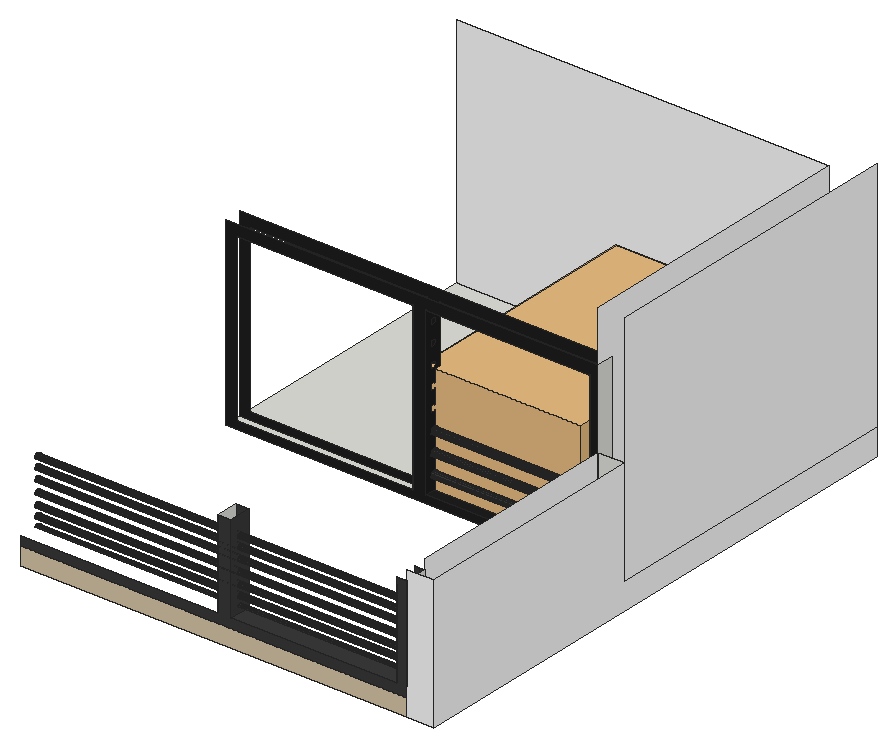
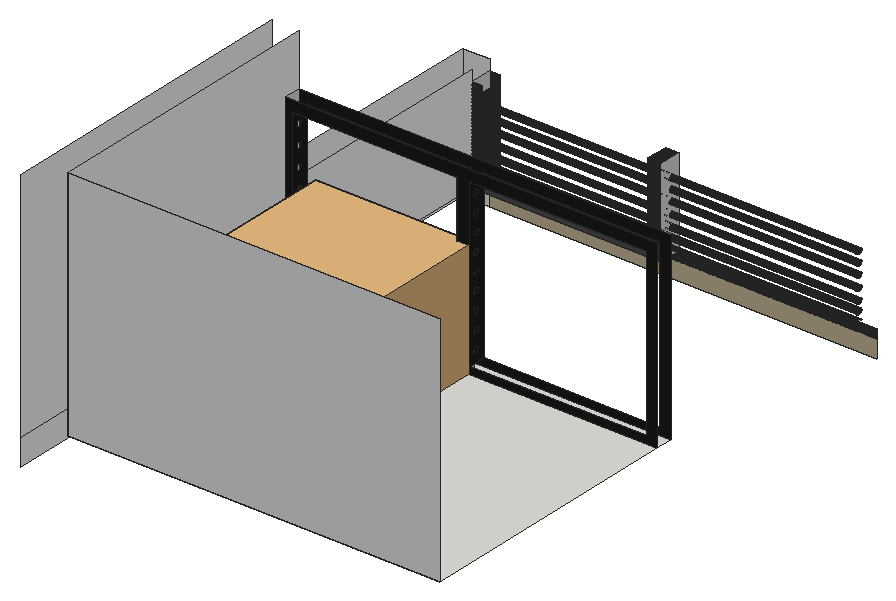
# SketchUp Ruby script. Lengths in inches.
U = 1.inch
M = Sketchup.active_model
def pt(a) = Geom::Point3d.new(a.map { |v| v * U })
def face(e, loops, mat)
  f = e.add_face(loops[0].map { |a| pt(a) })
  loops[1..].each { |l| e.add_face(l.map { |a| pt(a) }).erase! }
  f.material = f.back_material = mat if mat
  f
end
# faces: each face lists its corners as indices into pts; further lists are holes
def faces(e, pts, list, mat = nil) = list.each { |f| face(e, (f[0].is_a?(Array) ? f : [f]).map { |l| l.map { |i| pts[i] } }, mat) }
# xy, xz, yz: faces in a plane at the given z, y or x. An outline is a flat list of corners, or four numbers for a rectangle; further outlines are holes
def ring(l) = l.size == 4 ? [[l[0], l[1]], [l[2], l[1]], [l[2], l[3]], [l[0], l[3]]] : l.each_slice(2).to_a
def flat(e, list, mat, &to3) = list.each { |f| face(e, (f[0].is_a?(Array) ? f : [f]).map { |l| ring(l).map { |u, v| to3.(u, v) } }, mat) }
def xy(e, z, list, mat = nil) = flat(e, list, mat) { |x, y| [x, y, z] }
def xz(e, y, list, mat = nil) = flat(e, list, mat) { |x, z| [x, y, z] }
def yz(e, x, list, mat = nil) = flat(e, list, mat) { |y, z| [x, y, z] }
def lines(e, pts, list) = list.each { |a, b| e.add_line(pt(pts[a]), pt(pts[b])) }
# prism: a flat outline (further loops are holes) pulled along v
def prism(e, loops, v, mat = nil)
  f = face(e, loops, mat); d = Geom::Vector3d.new(v.map { |x| x * U })
  f.pushpull(f.normal.samedirection?(d) ? d.length : -d.length)
end
def box(e, o, s, mat = nil) = prism(e, [[o, [o[0] + s[0], o[1], o[2]], [o[0] + s[0], o[1] + s[1], o[2]], [o[0], o[1] + s[1], o[2]]]], [0, 0, s[2]], mat)
def at(x, y, z, deg = 0) = Geom::Transformation.translation(pt([x, y, z])) * Geom::Transformation.rotation(ORIGIN, Z_AXIS, deg.degrees)
def axes(o, x, y, z) = Geom::Transformation.new([*x, 0, *y, 0, *z, 0, *pt(o).to_a, 1])
def part(name) = M.definitions.add(name)
# library, detail: a bought-in or finely detailed component or shape, given as its bounding box
def library(name, o, s) = part(name).tap { |d| box(d.entities, o, s) }
def detail(e, o, s) = box(e.add_group.entities, o, s)
def put(e, d, t, mat = nil) = e.add_instance(d, t).tap { |i| i.material = mat if mat }
def group(e, t, mat = nil) = e.add_group.tap { |g| g.transformation = t; g.material = mat if mat }.entities
root = M.entities
M.materials.add("[Carrera Marble]").color = [252, 252, 252]
M.materials.add("[Color M07]").color = [58, 58, 58]
M.materials.add("[Color M08]").color = [30, 30, 30]
M.materials.add("[Field Square Tile]").color = [217, 201, 169]
M.materials.add("[Formica Laminate Dark]").color = [50, 53, 60]
c1 = library("2015 Porsche Macan",[0.14,0.6,0.32],[90.05,184.43,65.58])
xy(root,15.1875,[[467.61,406.29,679.23,416.16],[467.61,416.16,679.23,570.65]])
xy(root,15.1875,[[579.17,270.82,673.42,283.23]],"[Color M07]")
xy(root,19.3125,[[581.54,406.29,674.94,416.16]],"[Color M08]")
xz(root,270.82,[[679.23,0,694.52,75.25]],"[Carrera Marble]")
xz(root,270.82,[[459.28,9.82,679.23,9.82,679.23,69.375,673.42,69.375,673.42,15.1875,579.17,15.1875,579.17,65.34,571.61,65.34,571.61,15.1875,459.28,15.1875]],"[Color M07]")
xz(root,270.82,[[459.28,0,679.23,9.82]],"[Field Square Tile]")
xz(root,283.23,[[571.61,15.1875,579.17,65.34],[673.42,15.1875,675.77,69.375],[675.77,15.1875,679.23,69.375]],"[Color M07]")
xz(root,406.29,[[679.23,15.1875,694.52,75.25]])
xz(root,406.29,[[[467.61,15.1875,679.23,119.75],[473.77,19.3125,574.36,113.6],[581.54,19.3125,674.94,113.6]]],"[Color M08]")
xz(root,416.16,[[[467.61,15.1875,679.23,119.75],[473.77,19.3125,574.36,113.6],[581.54,19.3125,674.94,113.6]]],"[Color M08]")
xz(root,570.65,[[467.61,15.1875,679.23,149.125]],"[Carrera Marble]")
yz(root,571.61,[[270.82,15.1875,283.23,65.34]])
yz(root,574.36,[[[406.29,19.3125,416.16,113.6],[411.5,83.75,412,83.8125,412.47,84.01,412.87,84.32,413.18,84.72,413.37,85.18,413.4375,85.6875,413.37,86.1875,413.18,86.65,412.87,87.06,412.47,87.36,412,87.56,411.5,87.625,411,87.56,410.53,87.36,410.13,87.06,409.82,86.65,409.63,86.1875,409.5625,85.6875,409.63,85.18,409.82,84.72,410.13,84.32,410.53,84.01,411,83.8125],[411.5,73.75,412,73.8125,412.47,74.01,412.87,74.32,413.18,74.72,413.37,75.18,413.4375,75.6875,413.37,76.1875,413.18,76.65,412.87,77.06,412.47,77.36,412,77.56,411.5,77.625,411,77.56,410.53,77.36,410.13,77.06,409.82,76.65,409.63,76.1875,409.5625,75.6875,409.63,75.18,409.82,74.72,410.13,74.32,410.53,74.01,411,73.8125],[411.5,63.75,412,63.8125,412.47,64.01,412.87,64.32,413.18,64.72,413.37,65.18,413.4375,65.6875,413.37,66.1875,413.18,66.65,412.87,67.06,412.47,67.36,412,67.56,411.5,67.625,411,67.56,410.53,67.36,410.13,67.06,409.82,66.65,409.63,66.1875,409.5625,65.6875,409.63,65.18,409.82,64.72,410.13,64.32,410.53,64.01,411,63.8125],[411.5,53.75,412,53.8125,412.47,54.01,412.87,54.32,413.18,54.72,413.37,55.18,413.4375,55.6875,413.37,56.1875,413.18,56.65,412.87,57.06,412.47,57.36,412,57.56,411.5,57.625,411,57.56,410.53,57.36,410.13,57.06,409.82,56.65,409.63,56.1875,409.5625,55.6875,409.63,55.18,409.82,54.72,410.13,54.32,410.53,54.01,411,53.8125],[411.5,43.75,412,43.8125,412.47,44.01,412.87,44.32,413.18,44.72,413.37,45.18,413.4375,45.6875,413.37,46.1875,413.18,46.65,412.87,47.06,412.47,47.36,412,47.56,411.5,47.625,411,47.56,410.53,47.36,410.13,47.06,409.82,46.65,409.63,46.1875,409.5625,45.6875,409.63,45.18,409.82,44.72,410.13,44.32,410.53,44.01,411,43.8125],[411.5,33.75,412,33.8125,412.47,34.01,412.87,34.32,413.18,34.72,413.37,35.18,413.4375,35.6875,413.37,36.1875,413.18,36.65,412.87,37.06,412.47,37.36,412,37.56,411.5,37.625,411,37.56,410.53,37.36,410.13,37.06,409.82,36.65,409.63,36.1875,409.5625,35.6875,409.63,35.18,409.82,34.72,410.13,34.32,410.53,34.01,411,33.8125],[411.5,23.75,412,23.8125,412.47,24.01,412.87,24.32,413.18,24.72,413.37,25.18,413.4375,25.6875,413.37,26.1875,413.18,26.65,412.87,27.06,412.47,27.36,412,27.56,411.5,27.625,411,27.56,410.53,27.36,410.13,27.06,409.82,26.65,409.63,26.1875,409.5625,25.6875,409.63,25.18,409.82,24.72,410.13,24.32,410.53,24.01,411,23.8125],[411.5,103.75,412,103.8125,412.47,104.01,412.87,104.32,413.18,104.72,413.37,105.18,413.4375,105.6875,413.37,106.1875,413.18,106.65,412.87,107.06,412.47,107.36,412,107.56,411.5,107.625,411,107.56,410.53,107.36,410.13,107.06,409.82,106.65,409.63,106.1875,409.5625,105.6875,409.63,105.18,409.82,104.72,410.13,104.32,410.53,104.01,411,103.8125],[411.5,93.75,412,93.8125,412.47,94.01,412.87,94.32,413.18,94.72,413.37,95.18,413.4375,95.6875,413.37,96.1875,413.18,96.65,412.87,97.06,412.47,97.36,412,97.56,411.5,97.625,411,97.56,410.53,97.36,410.13,97.06,409.82,96.65,409.63,96.1875,409.5625,95.6875,409.63,95.18,409.82,94.72,410.13,94.32,410.53,94.01,411,93.8125]]],"[Color M08]")
yz(root,579.17,[[270.82,15.1875,283.23,65.34]],"[Color M07]")
yz(root,581.54,[[[406.29,19.3125,416.16,113.6],[411.43,103.83,410.92,103.9,410.46,104.09,410.06,104.4,409.75,104.8,409.55,105.27,409.49,105.77,409.55,106.27,409.75,106.74,410.06,107.14,410.46,107.45,410.92,107.64,411.43,107.71,411.93,107.64,412.39,107.45,412.8,107.14,413.1,106.74,413.3,106.27,413.36,105.77,413.3,105.27,413.1,104.8,412.8,104.4,412.39,104.09,411.93,103.9],[411.43,92.71,410.92,92.77,410.46,92.97,410.06,93.27,409.75,93.68,409.55,94.14,409.49,94.64,409.55,95.15,409.75,95.61,410.06,96.01,410.46,96.32,410.92,96.52,411.43,96.58,411.93,96.52,412.39,96.32,412.8,96.01,413.1,95.61,413.3,95.15,413.36,94.64,413.3,94.14,413.1,93.68,412.8,93.27,412.39,92.97,411.93,92.77],[411.43,81.58,410.92,81.65,410.46,81.84,410.06,82.15,409.75,82.55,409.55,83.02,409.49,83.52,409.55,84.02,409.75,84.49,410.06,84.89,410.46,85.2,410.92,85.39,411.43,85.46,411.93,85.39,412.39,85.2,412.8,84.89,413.1,84.49,413.3,84.02,413.36,83.52,413.3,83.02,413.1,82.55,412.8,82.15,412.39,81.84,411.93,81.65],[411.43,25.96,410.92,26.02,410.46,26.22,410.06,26.52,409.75,26.93,409.55,27.39,409.49,27.89,409.55,28.4,409.75,28.86,410.06,29.26,410.46,29.57,410.92,29.77,411.43,29.83,411.93,29.77,412.39,29.57,412.8,29.26,413.1,28.86,413.3,28.4,413.36,27.89,413.3,27.39,413.1,26.93,412.8,26.52,412.39,26.22,411.93,26.02],[411.43,37.08,410.92,37.15,410.46,37.34,410.06,37.65,409.75,38.05,409.55,38.52,409.49,39.02,409.55,39.52,409.75,39.99,410.06,40.39,410.46,40.7,410.92,40.89,411.43,40.96,411.93,40.89,412.39,40.7,412.8,40.39,413.1,39.99,413.3,39.52,413.36,39.02,413.3,38.52,413.1,38.05,412.8,37.65,412.39,37.34,411.93,37.15],[411.43,48.21,410.92,48.27,410.46,48.47,410.06,48.77,409.75,49.18,409.55,49.64,409.49,50.14,409.55,50.65,409.75,51.11,410.06,51.51,410.46,51.82,410.92,52.02,411.43,52.08,411.93,52.02,412.39,51.82,412.8,51.51,413.1,51.11,413.3,50.65,413.36,50.14,413.3,49.64,413.1,49.18,412.8,48.77,412.39,48.47,411.93,48.27],[411.43,70.46,410.92,70.52,410.46,70.72,410.06,71.02,409.75,71.43,409.55,71.89,409.49,72.39,409.55,72.9,409.75,73.36,410.06,73.76,410.46,74.07,410.92,74.27,411.43,74.33,411.93,74.27,412.39,74.07,412.8,73.76,413.1,73.36,413.3,72.9,413.36,72.39,413.3,71.89,413.1,71.43,412.8,71.02,412.39,70.72,411.93,70.52],[411.43,59.33,410.92,59.4,410.46,59.59,410.06,59.9,409.75,60.3,409.55,60.77,409.49,61.27,409.55,61.77,409.75,62.24,410.06,62.64,410.46,62.95,410.92,63.14,411.43,63.21,411.93,63.14,412.39,62.95,412.8,62.64,413.1,62.24,413.3,61.77,413.36,61.27,413.3,60.77,413.1,60.3,412.8,59.9,412.39,59.59,411.93,59.4]]],"[Color M08]")
yz(root,673.42,[[[270.82,15.1875,283.23,65.34],[276.43,23.27,276.8,23.32,277.15,23.46,277.44,23.6875,277.67,23.99,277.82,24.33,277.87,24.7,277.82,25.08,277.67,25.42,277.44,25.72,277.15,25.95,276.8,26.09,276.43,26.14,276.06,26.09,275.71,25.95,275.41,25.72,275.18,25.42,275.04,25.08,274.99,24.7,275.04,24.33,275.18,23.99,275.41,23.6875,275.71,23.46,276.06,23.32],[276.43,48.08,276.8,48.13,277.15,48.27,277.44,48.5,277.67,48.8,277.82,49.14,277.87,49.52,277.82,49.89,277.67,50.24,277.44,50.53,277.15,50.76,276.8,50.9,276.43,50.95,276.06,50.9,275.71,50.76,275.41,50.53,275.18,50.24,275.04,49.89,274.99,49.52,275.04,49.14,275.18,48.8,275.41,48.5,275.71,48.27,276.06,48.13],[276.43,41.89,276.8,41.94,277.15,42.08,277.44,42.3125,277.67,42.61,277.82,42.96,277.87,43.33,277.82,43.7,277.67,44.05,277.44,44.35,277.15,44.57,276.8,44.72,276.43,44.77,276.06,44.72,275.71,44.57,275.41,44.35,275.18,44.05,275.04,43.7,274.99,43.33,275.04,42.96,275.18,42.61,275.41,42.3125,275.71,42.08,276.06,41.94],[276.43,35.2,276.8,35.25,277.15,35.4,277.44,35.625,277.67,35.92,277.82,36.27,277.87,36.64,277.82,37.01,277.67,37.36,277.44,37.66,277.15,37.89,276.8,38.03,276.43,38.08,276.06,38.03,275.71,37.89,275.41,37.66,275.18,37.36,275.04,37.01,274.99,36.64,275.04,36.27,275.18,35.92,275.41,35.625,275.71,35.4,276.06,35.25],[276.43,28.77,276.8,28.82,277.15,28.96,277.44,29.1875,277.67,29.49,277.82,29.83,277.87,30.2,277.82,30.58,277.67,30.92,277.44,31.22,277.15,31.45,276.8,31.59,276.43,31.64,276.06,31.59,275.71,31.45,275.41,31.22,275.18,30.92,275.04,30.58,274.99,30.2,275.04,29.83,275.18,29.49,275.41,29.1875,275.71,28.96,276.06,28.82],[276.43,17.77,276.8,17.82,277.15,17.96,277.44,18.1875,277.67,18.49,277.82,18.83,277.87,19.2,277.82,19.58,277.67,19.92,277.44,20.22,277.15,20.45,276.8,20.59,276.43,20.64,276.06,20.59,275.71,20.45,275.41,20.22,275.18,19.92,275.04,19.58,274.99,19.2,275.04,18.83,275.18,18.49,275.41,18.1875,275.71,17.96,276.06,17.82],[276.43,59.2,276.8,59.25,277.15,59.4,277.44,59.625,277.67,59.92,277.82,60.27,277.87,60.64,277.82,61.01,277.67,61.36,277.44,61.66,277.15,61.89,276.8,62.03,276.43,62.08,276.06,62.03,275.71,61.89,275.41,61.66,275.18,61.36,275.04,61.01,274.99,60.64,275.04,60.27,275.18,59.92,275.41,59.625,275.71,59.4,276.06,59.25],[276.43,53.89,276.8,53.94,277.15,54.08,277.44,54.3125,277.67,54.61,277.82,54.96,277.87,55.33,277.82,55.7,277.67,56.05,277.44,56.35,277.15,56.57,276.8,56.72,276.43,56.77,276.06,56.72,275.71,56.57,275.41,56.35,275.18,56.05,275.04,55.7,274.99,55.33,275.04,54.96,275.18,54.61,275.41,54.3125,275.71,54.08,276.06,53.94]]],"[Color M07]")
yz(root,674.94,[[411.43,25.96,411.93,26.02,412.39,26.22,412.8,26.52,413.1,26.93,413.3,27.39,413.36,27.89,413.3,28.4,413.1,28.86,412.8,29.26,412.39,29.57,411.93,29.77,411.43,29.83,410.92,29.77,410.46,29.57,410.06,29.26,409.75,28.86,409.55,28.4,409.49,27.89,409.55,27.39,409.75,26.93,410.06,26.52,410.46,26.22,410.92,26.02],[411.43,37.08,411.93,37.15,412.39,37.34,412.8,37.65,413.1,38.05,413.3,38.52,413.36,39.02,413.3,39.52,413.1,39.99,412.8,40.39,412.39,40.7,411.93,40.89,411.43,40.96,410.92,40.89,410.46,40.7,410.06,40.39,409.75,39.99,409.55,39.52,409.49,39.02,409.55,38.52,409.75,38.05,410.06,37.65,410.46,37.34,410.92,37.15],[411.43,48.21,411.93,48.27,412.39,48.47,412.8,48.77,413.1,49.18,413.3,49.64,413.36,50.14,413.3,50.65,413.1,51.11,412.8,51.51,412.39,51.82,411.93,52.02,411.43,52.08,410.92,52.02,410.46,51.82,410.06,51.51,409.75,51.11,409.55,50.65,409.49,50.14,409.55,49.64,409.75,49.18,410.06,48.77,410.46,48.47,410.92,48.27]])
yz(root,674.94,[[[406.29,19.3125,416.16,113.6],[411.43,103.83,411.93,103.9,412.39,104.09,412.8,104.4,413.1,104.8,413.3,105.27,413.36,105.77,413.3,106.27,413.1,106.74,412.8,107.14,412.39,107.45,411.93,107.64,411.43,107.71,410.92,107.64,410.46,107.45,410.06,107.14,409.75,106.74,409.55,106.27,409.49,105.77,409.55,105.27,409.75,104.8,410.06,104.4,410.46,104.09,410.92,103.9],[411.43,92.71,411.93,92.77,412.39,92.97,412.8,93.27,413.1,93.68,413.3,94.14,413.36,94.64,413.3,95.15,413.1,95.61,412.8,96.01,412.39,96.32,411.93,96.52,411.43,96.58,410.92,96.52,410.46,96.32,410.06,96.01,409.75,95.61,409.55,95.15,409.49,94.64,409.55,94.14,409.75,93.68,410.06,93.27,410.46,92.97,410.92,92.77],[411.43,81.58,411.93,81.65,412.39,81.84,412.8,82.15,413.1,82.55,413.3,83.02,413.36,83.52,413.3,84.02,413.1,84.49,412.8,84.89,412.39,85.2,411.93,85.39,411.43,85.46,410.92,85.39,410.46,85.2,410.06,84.89,409.75,84.49,409.55,84.02,409.49,83.52,409.55,83.02,409.75,82.55,410.06,82.15,410.46,81.84,410.92,81.65],[411.43,70.46,411.93,70.52,412.39,70.72,412.8,71.02,413.1,71.43,413.3,71.89,413.36,72.39,413.3,72.9,413.1,73.36,412.8,73.76,412.39,74.07,411.93,74.27,411.43,74.33,410.92,74.27,410.46,74.07,410.06,73.76,409.75,73.36,409.55,72.9,409.49,72.39,409.55,71.89,409.75,71.43,410.06,71.02,410.46,70.72,410.92,70.52],[411.43,59.33,411.93,59.4,412.39,59.59,412.8,59.9,413.1,60.3,413.3,60.77,413.36,61.27,413.3,61.77,413.1,62.24,412.8,62.64,412.39,62.95,411.93,63.14,411.43,63.21,410.92,63.14,410.46,62.95,410.06,62.64,409.75,62.24,409.55,61.77,409.49,61.27,409.55,60.77,409.75,60.3,410.06,59.9,410.46,59.59,410.92,59.4],[411.43,48.21,411.93,48.27,412.39,48.47,412.8,48.77,413.1,49.18,413.3,49.64,413.36,50.14,413.3,50.65,413.1,51.11,412.8,51.51,412.39,51.82,411.93,52.02,411.43,52.08,410.92,52.02,410.46,51.82,410.06,51.51,409.75,51.11,409.55,50.65,409.49,50.14,409.55,49.64,409.75,49.18,410.06,48.77,410.46,48.47,410.92,48.27],[411.43,37.08,411.93,37.15,412.39,37.34,412.8,37.65,413.1,38.05,413.3,38.52,413.36,39.02,413.3,39.52,413.1,39.99,412.8,40.39,412.39,40.7,411.93,40.89,411.43,40.96,410.92,40.89,410.46,40.7,410.06,40.39,409.75,39.99,409.55,39.52,409.49,39.02,409.55,38.52,409.75,38.05,410.06,37.65,410.46,37.34,410.92,37.15],[411.43,25.96,411.93,26.02,412.39,26.22,412.8,26.52,413.1,26.93,413.3,27.39,413.36,27.89,413.3,28.4,413.1,28.86,412.8,29.26,412.39,29.57,411.93,29.77,411.43,29.83,410.92,29.77,410.46,29.57,410.06,29.26,409.75,28.86,409.55,28.4,409.49,27.89,409.55,27.39,409.75,26.93,410.06,26.52,410.46,26.22,410.92,26.02]]],"[Color M08]")
yz(root,679.23,[[270.82,15.1875,283.23,69.375],[406.29,15.1875,416.16,119.75]])
yz(root,679.23,[[283.23,15.1875,406.29,75.25],[416.16,15.1875,416.16,119.75,406.29,119.75,406.29,149.125,570.65,149.125,570.65,15.1875]],"[Carrera Marble]")
yz(root,694.52,[[270.82,0,585.18,0,585.18,15.1875,406.29,15.1875,406.29,75.25,270.82,75.25],[406.29,15.1875,585.18,149.125]],"[Carrera Marble]")
p = [[464.36,275.18,19.92],[464.36,275.04,19.58],[673.42,275.04,19.58],[673.42,275.18,19.92],[464.36,277.82,19.58],[464.36,277.67,19.92],
  [673.42,277.67,19.92],[673.42,277.82,19.58],[464.36,275.41,20.22],[673.42,275.41,20.22],[464.36,277.44,20.22],[673.42,277.44,20.22],
  [464.36,275.71,20.45],[673.42,275.71,20.45],[464.36,277.15,20.45],[673.42,277.15,20.45],[464.36,276.06,20.59],[673.42,276.06,20.59],
  [464.36,276.8,20.59],[673.42,276.8,20.59],[464.36,276.43,20.64],[673.42,276.43,20.64],[464.36,275.71,23.46],[464.36,276.06,23.32],
  [673.42,276.06,23.32],[673.42,275.71,23.46],[464.36,276.43,23.27],[673.42,276.43,23.27],[464.36,276.8,23.32],[673.42,276.8,23.32],
  [464.36,277.15,23.46],[673.42,277.15,23.46],[464.36,275.41,23.6875],[673.42,275.41,23.6875],[464.36,277.44,23.6875],[673.42,277.44,23.6875],
  [464.36,275.18,23.99],[673.42,275.18,23.99],[464.36,277.67,23.99],[673.42,277.67,23.99],[464.36,275.04,24.33],[673.42,275.04,24.33],
  [464.36,277.82,24.33],[673.42,277.82,24.33],[464.36,274.99,24.7],[673.42,274.99,24.7],[464.36,277.87,24.7],[673.42,277.87,24.7],
  [464.36,275.04,25.08],[673.42,275.04,25.08],[464.36,277.82,25.08],[673.42,277.82,25.08],[464.36,275.18,25.42],[673.42,275.18,25.42],
  [464.36,277.67,25.42],[673.42,277.67,25.42],[464.36,275.41,25.72],[673.42,275.41,25.72],[464.36,277.44,25.72],[673.42,277.44,25.72],
  [464.36,275.71,25.95],[673.42,275.71,25.95],[464.36,277.15,25.95],[673.42,277.15,25.95],[464.36,276.06,26.09],[673.42,276.06,26.09],
  [464.36,276.8,26.09],[673.42,276.8,26.09],[674.94,410.92,26.02],[674.94,410.46,26.22],[581.54,410.46,26.22],[581.54,410.92,26.02],
  [674.94,411.43,25.96],[581.54,411.43,25.96],[674.94,411.93,26.02],[581.54,411.93,26.02],[674.94,412.39,26.22],[581.54,412.39,26.22],
  [464.36,276.43,26.14],[673.42,276.43,26.14],[674.94,410.06,26.52],[581.54,410.06,26.52],[674.94,412.8,26.52],[581.54,412.8,26.52],
  [674.94,409.75,26.93],[581.54,409.75,26.93],[674.94,413.1,26.93],[581.54,413.1,26.93],[674.94,409.55,27.39],[581.54,409.55,27.39],
  [674.94,413.3,27.39],[581.54,413.3,27.39],[674.94,409.49,27.89],[581.54,409.49,27.89],[674.94,413.36,27.89],[581.54,413.36,27.89],
  [674.94,409.55,28.4],[581.54,409.55,28.4],[674.94,413.3,28.4],[581.54,413.3,28.4],[674.94,409.75,28.86],[581.54,409.75,28.86],
  [674.94,413.1,28.86],[581.54,413.1,28.86],[464.36,275.71,28.96],[464.36,276.06,28.82],[673.42,276.06,28.82],[673.42,275.71,28.96],
  [464.36,276.43,28.77],[673.42,276.43,28.77],[464.36,276.8,28.82],[673.42,276.8,28.82],[464.36,277.15,28.96],[673.42,277.15,28.96],
  [674.94,410.06,29.26],[581.54,410.06,29.26],[674.94,412.8,29.26],[581.54,412.8,29.26],[464.36,275.41,29.1875],[673.42,275.41,29.1875],
  [464.36,277.44,29.1875],[673.42,277.44,29.1875],[464.36,275.18,29.49],[673.42,275.18,29.49],[464.36,277.67,29.49],[673.42,277.67,29.49],
  [674.94,410.46,29.57],[581.54,410.46,29.57],[674.94,412.39,29.57],[581.54,412.39,29.57],[464.36,275.04,29.83],[673.42,275.04,29.83],
  [464.36,277.82,29.83],[673.42,277.82,29.83],[674.94,410.92,29.77],[581.54,410.92,29.77],[674.94,411.93,29.77],[581.54,411.93,29.77],
  [464.36,274.99,30.2],[673.42,274.99,30.2],[464.36,277.87,30.2],[673.42,277.87,30.2],[674.94,411.43,29.83],[581.54,411.43,29.83],
  [464.36,275.04,30.58],[673.42,275.04,30.58],[464.36,277.82,30.58],[673.42,277.82,30.58],[464.36,275.18,30.92],[673.42,275.18,30.92],
  [464.36,277.67,30.92],[673.42,277.67,30.92],[464.36,275.41,31.22],[673.42,275.41,31.22],[464.36,277.44,31.22],[673.42,277.44,31.22],
  [464.36,275.71,31.45],[673.42,275.71,31.45],[464.36,277.15,31.45],[673.42,277.15,31.45],[464.36,276.06,31.59],[673.42,276.06,31.59],
  [464.36,276.8,31.59],[673.42,276.8,31.59],[464.36,276.43,31.64],[673.42,276.43,31.64],[464.36,276.06,35.25],[464.36,276.43,35.2],
  [673.42,276.43,35.2],[673.42,276.06,35.25],[464.36,276.8,35.25],[673.42,276.8,35.25],[464.36,275.71,35.4],[673.42,275.71,35.4],
  [464.36,277.15,35.4],[673.42,277.15,35.4],[464.36,275.41,35.625],[673.42,275.41,35.625],[464.36,277.44,35.625],[673.42,277.44,35.625],
  [464.36,275.18,35.92],[673.42,275.18,35.92],[464.36,277.67,35.92],[673.42,277.67,35.92],[464.36,275.04,36.27],[673.42,275.04,36.27],
  [464.36,277.82,36.27],[673.42,277.82,36.27],[464.36,274.99,36.64],[673.42,274.99,36.64],[464.36,277.87,36.64],[673.42,277.87,36.64],
  [464.36,275.04,37.01],[673.42,275.04,37.01],[464.36,277.82,37.01],[673.42,277.82,37.01],[464.36,275.18,37.36],[673.42,275.18,37.36],
  [464.36,277.67,37.36],[673.42,277.67,37.36],[674.94,410.92,37.15],[674.94,410.46,37.34],[581.54,410.46,37.34],[581.54,410.92,37.15],
  [674.94,411.43,37.08],[581.54,411.43,37.08],[674.94,411.93,37.15],[581.54,411.93,37.15],[674.94,412.39,37.34],[581.54,412.39,37.34],
  [674.94,410.06,37.65],[581.54,410.06,37.65],[674.94,412.8,37.65],[581.54,412.8,37.65],[464.36,275.41,37.66],[673.42,275.41,37.66],
  [464.36,277.44,37.66],[673.42,277.44,37.66],[674.94,409.75,38.05],[581.54,409.75,38.05],[674.94,413.1,38.05],[581.54,413.1,38.05],
  [464.36,275.71,37.89],[673.42,275.71,37.89],[464.36,277.15,37.89],[673.42,277.15,37.89],[464.36,276.06,38.03],[673.42,276.06,38.03],
  [464.36,276.8,38.03],[673.42,276.8,38.03],[464.36,276.43,38.08],[673.42,276.43,38.08],[674.94,409.55,38.52],[581.54,409.55,38.52],
  [674.94,413.3,38.52],[581.54,413.3,38.52],[674.94,409.49,39.02],[581.54,409.49,39.02],[674.94,413.36,39.02],[581.54,413.36,39.02],
  [674.94,409.55,39.52],[581.54,409.55,39.52],[674.94,413.3,39.52],[581.54,413.3,39.52],[674.94,409.75,39.99],[581.54,409.75,39.99],
  [674.94,413.1,39.99],[581.54,413.1,39.99],[674.94,410.06,40.39],[581.54,410.06,40.39],[674.94,412.8,40.39],[581.54,412.8,40.39],
  [674.94,410.46,40.7],[581.54,410.46,40.7],[674.94,412.39,40.7],[581.54,412.39,40.7],[674.94,410.92,40.89],[581.54,410.92,40.89],
  [674.94,411.93,40.89],[581.54,411.93,40.89],[674.94,411.43,40.96],[581.54,411.43,40.96],[464.36,275.71,42.08],[464.36,276.06,41.94],
  [673.42,276.06,41.94],[673.42,275.71,42.08],[464.36,276.43,41.89],[673.42,276.43,41.89],[464.36,276.8,41.94],[673.42,276.8,41.94],
  [464.36,277.15,42.08],[673.42,277.15,42.08],[464.36,275.41,42.3125],[673.42,275.41,42.3125],[464.36,277.44,42.3125],[673.42,277.44,42.3125],
  [464.36,275.18,42.61],[673.42,275.18,42.61],[464.36,277.67,42.61],[673.42,277.67,42.61],[464.36,275.04,42.96],[673.42,275.04,42.96],
  [464.36,277.82,42.96],[673.42,277.82,42.96],[464.36,274.99,43.33],[673.42,274.99,43.33],[464.36,277.87,43.33],[673.42,277.87,43.33],
  [464.36,275.04,43.7],[673.42,275.04,43.7],[464.36,277.82,43.7],[673.42,277.82,43.7],[464.36,275.18,44.05],[673.42,275.18,44.05],
  [464.36,277.67,44.05],[673.42,277.67,44.05],[464.36,275.41,44.35],[673.42,275.41,44.35],[464.36,277.44,44.35],[673.42,277.44,44.35],
  [464.36,275.71,44.57],[673.42,275.71,44.57],[464.36,277.15,44.57],[673.42,277.15,44.57],[464.36,276.06,44.72],[673.42,276.06,44.72],
  [464.36,276.8,44.72],[673.42,276.8,44.72],[464.36,276.43,44.77],[673.42,276.43,44.77],[464.36,275.71,48.27],[464.36,276.06,48.13],
  [673.42,276.06,48.13],[673.42,275.71,48.27],[464.36,276.43,48.08],[673.42,276.43,48.08],[464.36,276.8,48.13],[673.42,276.8,48.13],
  [464.36,277.15,48.27],[673.42,277.15,48.27],[674.94,411.43,48.21],[674.94,410.92,48.27],[581.54,410.92,48.27],[581.54,411.43,48.21],
  [674.94,411.93,48.27],[581.54,411.93,48.27],[464.36,275.41,48.5],[673.42,275.41,48.5],[464.36,277.44,48.5],[673.42,277.44,48.5],
  [674.94,410.46,48.47],[581.54,410.46,48.47],[674.94,412.39,48.47],[581.54,412.39,48.47],[464.36,275.18,48.8],[673.42,275.18,48.8],
  [464.36,277.67,48.8],[673.42,277.67,48.8],[674.94,410.06,48.77],[581.54,410.06,48.77],[674.94,412.8,48.77],[581.54,412.8,48.77],
  [464.36,275.04,49.14],[673.42,275.04,49.14],[464.36,277.82,49.14],[673.42,277.82,49.14],[674.94,409.75,49.18],[581.54,409.75,49.18],
  [674.94,413.1,49.18],[581.54,413.1,49.18],[464.36,274.99,49.52],[673.42,274.99,49.52],[464.36,277.87,49.52],[673.42,277.87,49.52],
  [674.94,409.55,49.64],[581.54,409.55,49.64],[674.94,413.3,49.64],[581.54,413.3,49.64],[464.36,275.04,49.89],[673.42,275.04,49.89],
  [464.36,277.82,49.89],[673.42,277.82,49.89],[674.94,409.49,50.14],[581.54,409.49,50.14],[674.94,413.36,50.14],[581.54,413.36,50.14],
  [464.36,275.18,50.24],[673.42,275.18,50.24],[464.36,277.67,50.24],[673.42,277.67,50.24],[674.94,409.55,50.65],[581.54,409.55,50.65],
  [674.94,413.3,50.65],[581.54,413.3,50.65],[464.36,275.41,50.53],[673.42,275.41,50.53],[464.36,277.44,50.53],[673.42,277.44,50.53],
  [464.36,275.71,50.76],[673.42,275.71,50.76],[464.36,277.15,50.76],[673.42,277.15,50.76],[674.94,409.75,51.11],[581.54,409.75,51.11],
  [674.94,413.1,51.11],[581.54,413.1,51.11],[464.36,276.06,50.9],[673.42,276.06,50.9],[464.36,276.8,50.9],[673.42,276.8,50.9],
  [464.36,276.43,50.95],[673.42,276.43,50.95],[674.94,410.06,51.51],[581.54,410.06,51.51],[674.94,412.8,51.51],[581.54,412.8,51.51],
  [674.94,410.46,51.82],[581.54,410.46,51.82],[674.94,412.39,51.82],[581.54,412.39,51.82],[674.94,410.92,52.02],[581.54,410.92,52.02],
  [674.94,411.93,52.02],[581.54,411.93,52.02],[674.94,411.43,52.08],[581.54,411.43,52.08],[464.36,275.71,54.08],[464.36,276.06,53.94],
  [673.42,276.06,53.94],[673.42,275.71,54.08],[464.36,276.43,53.89],[673.42,276.43,53.89],[464.36,276.8,53.94],[673.42,276.8,53.94],
  [464.36,277.15,54.08],[673.42,277.15,54.08],[464.36,275.41,54.3125],[673.42,275.41,54.3125],[464.36,277.44,54.3125],[673.42,277.44,54.3125],
  [464.36,275.18,54.61],[673.42,275.18,54.61],[464.36,277.67,54.61],[673.42,277.67,54.61],[464.36,275.04,54.96],[673.42,275.04,54.96],
  [464.36,277.82,54.96],[673.42,277.82,54.96],[464.36,274.99,55.33],[673.42,274.99,55.33],[464.36,277.87,55.33],[673.42,277.87,55.33],
  [464.36,275.04,55.7],[673.42,275.04,55.7],[464.36,277.82,55.7],[673.42,277.82,55.7],[464.36,275.18,56.05],[673.42,275.18,56.05],
  [464.36,277.67,56.05],[673.42,277.67,56.05],[464.36,275.41,56.35],[673.42,275.41,56.35],[464.36,277.44,56.35],[673.42,277.44,56.35],
  [464.36,275.71,56.57],[673.42,275.71,56.57],[464.36,277.15,56.57],[673.42,277.15,56.57],[464.36,276.06,56.72],[673.42,276.06,56.72],
  [464.36,276.8,56.72],[673.42,276.8,56.72],[464.36,276.43,56.77],[673.42,276.43,56.77]]
faces(root,p,[[0,1,2,3],[4,5,6,7],[8,0,3,9],[5,10,11,6],[12,8,9,13],[10,14,15,11],[16,12,13,17],[14,18,19,15],
  [20,16,17,21],[18,20,21,19],[22,23,24,25],[23,26,27,24],[26,28,29,27],[28,30,31,29],[32,22,25,33],[30,34,35,31],
  [36,32,33,37],[34,38,39,35],[40,36,37,41],[38,42,43,39],[44,40,41,45],[42,46,47,43],[48,44,45,49],[46,50,51,47],
  [52,48,49,53],[50,54,55,51],[56,52,53,57],[54,58,59,55],[60,56,57,61],[58,62,63,59],[64,60,61,65],[62,66,67,63],
  [78,64,65,79],[66,78,79,67],[104,105,106,107],[105,108,109,106],[108,110,111,109],[110,112,113,111],[118,104,107,119],[112,120,121,113],
  [122,118,119,123],[120,124,125,121],[130,122,123,131],[124,132,133,125],[138,130,131,139],[132,140,141,133],[144,138,139,145],[140,146,147,141],
  [148,144,145,149],[146,150,151,147],[152,148,149,153],[150,154,155,151],[156,152,153,157],[154,158,159,155],[160,156,157,161],[158,162,163,159],
  [164,160,161,165],[162,164,165,163],[166,167,168,169],[167,170,171,168],[172,166,169,173],[170,174,175,171],[176,172,173,177],[174,178,179,175],
  [180,176,177,181],[178,182,183,179],[184,180,181,185],[182,186,187,183],[188,184,185,189],[186,190,191,187],[192,188,189,193],[190,194,195,191],
  [196,192,193,197],[194,198,199,195],[214,196,197,215],[198,216,217,199],[222,214,215,223],[216,224,225,217],[226,222,223,227],[224,228,229,225],
  [230,226,227,231],[228,230,231,229],[262,263,264,265],[263,266,267,264],[266,268,269,267],[268,270,271,269],[272,262,265,273],[270,274,275,271],
  [276,272,273,277],[274,278,279,275],[280,276,277,281],[278,282,283,279],[284,280,281,285],[282,286,287,283],[288,284,285,289],[286,290,291,287],
  [292,288,289,293],[290,294,295,291],[296,292,293,297],[294,298,299,295],[300,296,297,301],[298,302,303,299],[304,300,301,305],[302,306,307,303],
  [308,304,305,309],[306,308,309,307],[310,311,312,313],[311,314,315,312],[314,316,317,315],[316,318,319,317],[326,310,313,327],[318,328,329,319],
  [334,326,327,335],[328,336,337,329],[342,334,335,343],[336,344,345,337],[350,342,343,351],[344,352,353,345],[358,350,351,359],[352,360,361,353],
  [366,358,359,367],[360,368,369,361],[374,366,367,375],[368,376,377,369],[378,374,375,379],[376,380,381,377],[386,378,379,387],[380,388,389,381],
  [390,386,387,391],[388,390,391,389],[406,407,408,409],[407,410,411,408],[410,412,413,411],[412,414,415,413],[416,406,409,417],[414,418,419,415],
  [420,416,417,421],[418,422,423,419],[424,420,421,425],[422,426,427,423],[428,424,425,429],[426,430,431,427],[432,428,429,433],[430,434,435,431],
  [436,432,433,437],[434,438,439,435],[440,436,437,441],[438,442,443,439],[444,440,441,445],[442,446,447,443],[448,444,445,449],[446,450,451,447],
  [452,448,449,453],[450,452,453,451]],"[Formica Laminate Dark]")
faces(root,p,[[68,69,70,71],[72,68,71,73],[74,72,73,75],[76,74,75,77],[69,80,81,70],[82,76,77,83],[80,84,85,81],[86,82,83,87],
  [84,88,89,85],[90,86,87,91],[88,92,93,89],[94,90,91,95],[92,96,97,93],[98,94,95,99],[96,100,101,97],[102,98,99,103],
  [100,114,115,101],[116,102,103,117],[114,126,127,115],[128,116,117,129],[126,134,135,127],[136,128,129,137],[134,142,143,135],[142,136,137,143],
  [200,201,202,203],[204,200,203,205],[206,204,205,207],[208,206,207,209],[201,210,211,202],[212,208,209,213],[210,218,219,211],[220,212,213,221],
  [218,232,233,219],[234,220,221,235],[232,236,237,233],[238,234,235,239],[236,240,241,237],[242,238,239,243],[240,244,245,241],[246,242,243,247],
  [244,248,249,245],[250,246,247,251],[248,252,253,249],[254,250,251,255],[252,256,257,253],[258,254,255,259],[256,260,261,257],[260,258,259,261],
  [320,321,322,323],[324,320,323,325],[321,330,331,322],[332,324,325,333],[330,338,339,331],[340,332,333,341],[338,346,347,339],[348,340,341,349],
  [346,354,355,347],[356,348,349,357],[354,362,363,355],[364,356,357,365],[362,370,371,363],[372,364,365,373],[370,382,383,371],[384,372,373,385],
  [382,392,393,383],[394,384,385,395],[392,396,397,393],[398,394,395,399],[396,400,401,397],[402,398,399,403],[400,404,405,401],[404,402,403,405]],"[Color M07]")
put(root,c1,axes([574.49,412.17,15.1875],[1,0,0],[0,0.7462,0],[0,0,1]))
